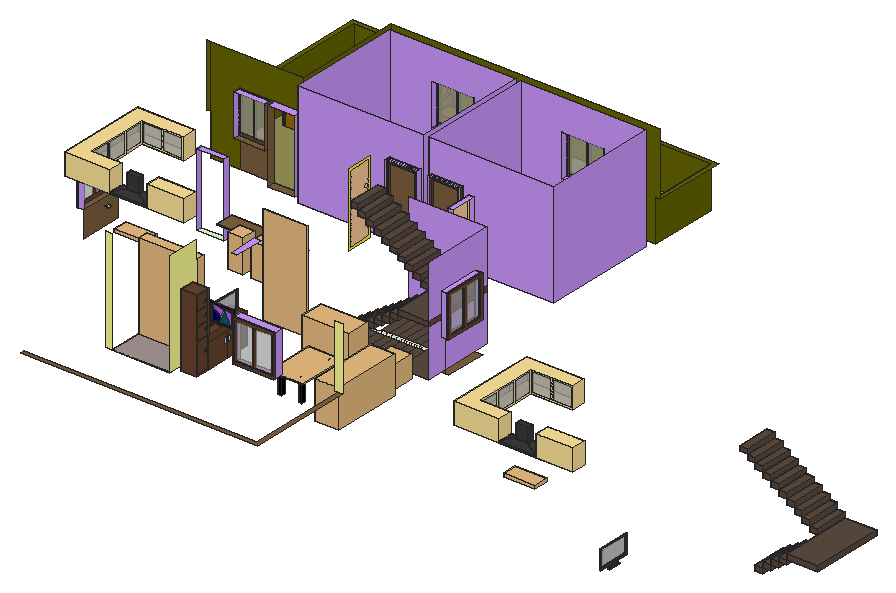
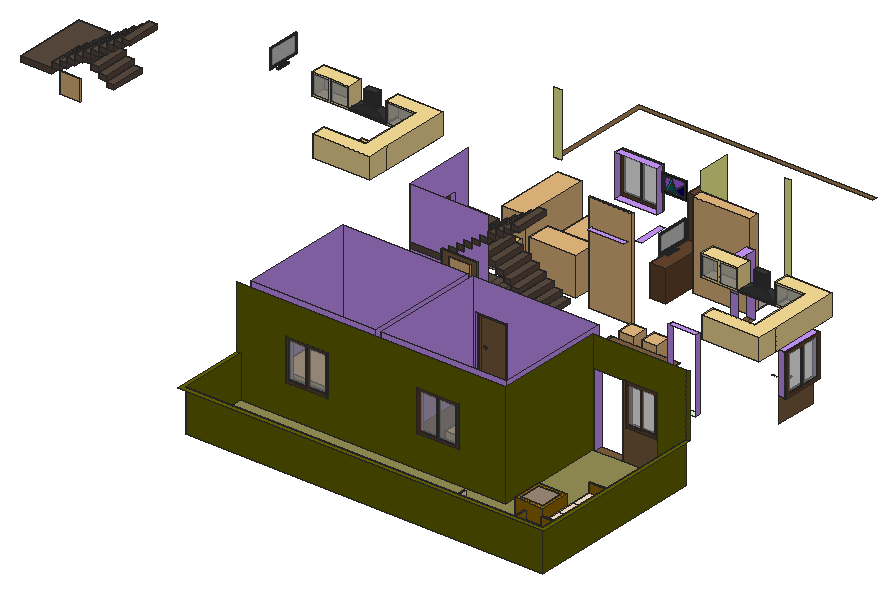
# SketchUp Ruby script. Lengths in inches.
U = 1.inch
M = Sketchup.active_model
def pt(a) = Geom::Point3d.new(a.map { |v| v * U })
def face(e, loops, mat)
  f = e.add_face(loops[0].map { |a| pt(a) })
  loops[1..].each { |l| e.add_face(l.map { |a| pt(a) }).erase! }
  f.material = f.back_material = mat if mat
  f
end
# faces: each face lists its corners as indices into pts; further lists are holes
def faces(e, pts, list, mat = nil) = list.each { |f| face(e, (f[0].is_a?(Array) ? f : [f]).map { |l| l.map { |i| pts[i] } }, mat) }
# xy, xz, yz: faces in a plane at the given z, y or x. An outline is a flat list of corners, or four numbers for a rectangle; further outlines are holes
def ring(l) = l.size == 4 ? [[l[0], l[1]], [l[2], l[1]], [l[2], l[3]], [l[0], l[3]]] : l.each_slice(2).to_a
def flat(e, list, mat, &to3) = list.each { |f| face(e, (f[0].is_a?(Array) ? f : [f]).map { |l| ring(l).map { |u, v| to3.(u, v) } }, mat) }
def xy(e, z, list, mat = nil) = flat(e, list, mat) { |x, y| [x, y, z] }
def xz(e, y, list, mat = nil) = flat(e, list, mat) { |x, z| [x, y, z] }
def yz(e, x, list, mat = nil) = flat(e, list, mat) { |y, z| [x, y, z] }
def lines(e, pts, list) = list.each { |a, b| e.add_line(pt(pts[a]), pt(pts[b])) }
# prism: a flat outline (further loops are holes) pulled along v
def prism(e, loops, v, mat = nil)
  f = face(e, loops, mat); d = Geom::Vector3d.new(v.map { |x| x * U })
  f.pushpull(f.normal.samedirection?(d) ? d.length : -d.length)
end
def box(e, o, s, mat = nil) = prism(e, [[o, [o[0] + s[0], o[1], o[2]], [o[0] + s[0], o[1] + s[1], o[2]], [o[0], o[1] + s[1], o[2]]]], [0, 0, s[2]], mat)
def at(x, y, z, deg = 0) = Geom::Transformation.translation(pt([x, y, z])) * Geom::Transformation.rotation(ORIGIN, Z_AXIS, deg.degrees)
def axes(o, x, y, z) = Geom::Transformation.new([*x, 0, *y, 0, *z, 0, *pt(o).to_a, 1])
def part(name) = M.definitions.add(name)
# library, detail: a bought-in or finely detailed component or shape, given as its bounding box
def library(name, o, s) = part(name).tap { |d| box(d.entities, o, s) }
def detail(e, o, s) = box(e.add_group.entities, o, s)
def put(e, d, t, mat = nil) = e.add_instance(d, t).tap { |i| i.material = mat if mat }
def group(e, t, mat = nil) = e.add_group.tap { |g| g.transformation = t; g.material = mat if mat }.entities
root = M.entities
M.materials.add("C01_Vanilla_Cream").color = [255, 230, 206]
M.materials.add("C02_Golden_Beige").color = [255, 205, 155]
M.materials.add("D02_Buttercup_Glow").color = [255, 229, 155]
M.materials.add("D07_Ochre_Flame").color = [153, 107, 0]
M.materials.add("E01_Mint_Frost").color = [255, 255, 204]
M.materials.add("E02_Pale_Lime").color = [255, 255, 153]
M.materials.add("E04_Green_Bloom").color = [255, 255, 49]
M.materials.add("E08_Lime_Depth").color = [102, 102, 0]
M.materials.add("F06_Grassy_Shade").color = [102, 204, 0]
M.materials.add("G07_Jungle_Burst").color = [0, 153, 0]
M.materials.add("Glass_Mirror_01").color = [185, 185, 185]
M.materials["Glass_Mirror_01"].alpha = 0.91
M.materials.add("Glass_Mirror_2").color = [185, 185, 185]
M.materials["Glass_Mirror_2"].alpha = 0.8
M.materials.add("Glass_Mirror_3").color = [185, 185, 185]
M.materials["Glass_Mirror_3"].alpha = 0.65
M.materials.add("Glass_Mirror_4").color = [185, 185, 185]
M.materials["Glass_Mirror_4"].alpha = 0.68
M.materials.add("Glass_Sky Reflection_01").color = [126, 138, 183]
M.materials["Glass_Sky Reflection_01"].alpha = 0.25
M.materials.add("H06_Ocean_Depth").color = [0, 204, 204]
M.materials.add("H08_Emerald_Abyss").color = [0, 102, 102]
M.materials.add("I03_Bluebell_Mist").color = [101, 101, 255]
M.materials.add("I08_Inkstorm").color = [0, 0, 102]
M.materials.add("J02_Lavender_Veil").color = [204, 153, 255]
M.materials.add("J03_Orchid_Glow").color = [178, 101, 255]
M.materials.add("K02_Rosy_Glow").color = [255, 153, 255]
M.materials.add("M07_Charcoal_Gleam").color = [58, 58, 58]
M.materials.add("M09_Shadow_Night").color = [0, 0, 0]
M.materials.add("Marble_01_1K").color = [230, 255, 211]
M.materials.add("Marble_03_1K").color = [175, 182, 201]
M.materials.add("Marble_06_1K").color = [165, 150, 147]
M.materials.add("Marble_07_1K").color = [36, 34, 36]
M.materials.add("Marble_20_1K").color = [172, 173, 182]
M.materials.add("Metal_06_1K").color = [238, 236, 231]
M.materials.add("Plaster_02_1K").color = [157, 140, 119]
M.materials.add("Plywood_01_1K").color = [125, 96, 64]
M.materials.add("Soil_04_1K").color = [152, 146, 88]
M.materials.add("Wood_Floor_12_1K").color = [92, 75, 65]
M.materials.add("Wood_Veneer_15_1K").color = [103, 69, 45]
c1 = part("Group\#70")
box(c1.entities,[0,0,0],[9,39,6],"Wood_Floor_12_1K")
c2 = part("Group\#38")
xy(c2.entities,0,[[67.3125,0,69.625,27.1875],[-2.33,24.1875,67.3125,27.1875]],"D07_Ochre_Flame")
xy(c2.entities,18.3125,[[0,0,22.82,24.1875],[22.82,0,45.07,24.1875],[45.07,0,67.3125,24.1875]],"C01_Vanilla_Cream")
xy(c2.entities,24.5625,[[67.3125,0,69.625,27.1875]],"D07_Ochre_Flame")
xy(c2.entities,28.6875,[[-2.33,0,0,24.1875]],"D07_Ochre_Flame")
xy(c2.entities,33.375,[[-2.33,24.1875,67.3125,27.1875]],"D07_Ochre_Flame")
xz(c2.entities,0,[[0,0,22.82,18.3125],[22.82,0,45.07,18.3125],[45.07,0,67.3125,18.3125]],"C01_Vanilla_Cream")
xz(c2.entities,0,[[-2.33,0,0,28.6875],[67.3125,0,69.625,24.5625]],"D07_Ochre_Flame")
xz(c2.entities,24.1875,[[-2.33,0,67.3125,0,67.3125,18.3125,0,18.3125,0,28.6875,-2.33,28.6875],[0,18.3125,22.82,33.375],[22.82,18.3125,45.07,33.375],[45.07,18.3125,67.3125,33.375],[-2.33,28.6875,0,33.375]],"D07_Ochre_Flame")
xz(c2.entities,27.1875,[[-2.33,0,67.3125,33.375],[67.3125,0,69.625,24.5625]],"D07_Ochre_Flame")
yz(c2.entities,-2.33,[[0,0,24.1875,28.6875],[24.1875,0,27.1875,33.375]],"D07_Ochre_Flame")
yz(c2.entities,0,[[0,18.3125,24.1875,28.6875]],"D07_Ochre_Flame")
yz(c2.entities,67.3125,[[0,0,24.1875,18.3125],[0,18.3125,24.1875,24.5625]],"C01_Vanilla_Cream")
yz(c2.entities,67.3125,[[24.1875,0,27.1875,24.5625],[24.1875,24.5625,27.1875,33.375]],"D07_Ochre_Flame")
yz(c2.entities,69.625,[[0,0,27.1875,24.5625]],"D07_Ochre_Flame")
c3 = part("Group\#43")
box(c3.entities,[0,0,0],[1,4.5625,0.25],"Metal_06_1K")
c4 = part("Group\#42")
xy(c4.entities,0,[[0,-1.93,40.35,0],[0,0,40.35,21.25]],"Plywood_01_1K")
xy(c4.entities,25.125,[[0,0,40.35,21.25]],"Marble_07_1K")
xy(c4.entities,25.1875,[[20.85,8.75,21.39,8.86,21.89,9.11,22.3,9.47,22.61,9.94,22.79,10.46,22.82,11.01,22.71,11.56,22.47,12.06,22.1,12.47,21.64,12.78,21.11,12.96,20.56,12.99,20.01,12.88,19.52,12.63,19.1,12.27,18.79,11.81,18.62,11.28,18.58,10.73,18.69,10.18,18.9375,9.69,19.31,9.27,19.77,8.96,20.29,8.79]],"M09_Shadow_Night")
xy(c4.entities,25.1875,[[[8.8,4,31.8,17.68],[20.85,8.75,20.29,8.79,19.77,8.96,19.31,9.27,18.9375,9.69,18.69,10.18,18.58,10.73,18.62,11.28,18.79,11.81,19.1,12.27,19.52,12.63,20.01,12.88,20.56,12.99,21.11,12.96,21.64,12.78,22.1,12.47,22.47,12.06,22.71,11.56,22.82,11.01,22.79,10.46,22.61,9.94,22.3,9.47,21.89,9.11,21.39,8.86]]],"Marble_07_1K")
xy(c4.entities,26,[[0,-1.93,40.35,0]],"Plywood_01_1K")
xy(c4.entities,26.5625,[[[0,0,40.35,21.25],[8.8,4,31.8,17.68]]],"Marble_07_1K")
xy(c4.entities,71.66,[[0,-1.93,40.35,0]],"Plywood_01_1K")
xz(c4.entities,-1.93,[[0,0,40.35,26],[0,26,40.35,71.66]],"Plywood_01_1K")
xz(c4.entities,0,[[0,25.125,40.35,26],[0,26,40.35,26.5625]],"Marble_07_1K")
xz(c4.entities,0,[[0,0,40.35,25.125],[0,26.5625,40.35,71.66]],"Plywood_01_1K")
xz(c4.entities,4,[[8.8,25.1875,31.8,26.5625]],"Marble_07_1K")
xz(c4.entities,17.68,[[8.8,25.1875,31.8,26.5625]],"Marble_07_1K")
xz(c4.entities,21.25,[[0,25.125,40.35,26.5625]],"Marble_07_1K")
xz(c4.entities,21.25,[[0,0,20.17,21],[20.17,0,40.35,21],[0,21,40.35,25.125]],"Plywood_01_1K")
yz(c4.entities,0,[[0,25.125,21.25,26.5625]],"Marble_07_1K")
yz(c4.entities,0,[[-1.93,0,0,26],[0,0,21.25,25.125],[-1.93,26,0,71.66]],"Plywood_01_1K")
yz(c4.entities,8.8,[[4,25.1875,17.68,26.5625]],"Marble_07_1K")
yz(c4.entities,31.8,[[4,25.1875,17.68,26.5625]],"Marble_07_1K")
yz(c4.entities,40.35,[[0,25.125,21.25,26.5625]],"Marble_07_1K")
yz(c4.entities,40.35,[[-1.93,0,0,26],[0,0,21.25,25.125],[-1.93,26,0,71.66]],"Plywood_01_1K")
put(c4.entities,c3,axes([22.63,21.25,13.17],[-1,0,0],[0,0,1],[0,1,0]))
put(c4.entities,c3,axes([18.69,21.25,13.17],[-1,0,0],[0,0,1],[0,1,0]))
put(c4.entities,c3,axes([22.61,21.25,24.2],[0,0,-1],[-1,0,0],[0,1,0]))
c5 = part("Group\#15")
box(c5.entities,[0,0,0],[4,4,24])
c6 = part("Group\#47")
box(c6.entities,[0,0,0],[65.6875,38.91,0.4375],"Marble_06_1K")
c7 = part("Group\#10")
detail(c7.entities,[0,-4,0],[28,80,43.625])
c8 = part("Group\#14")
box(c8.entities,[0,0,0],[4,4,24])
c9 = part("Group\#29")
box(c9.entities,[0,0,0],[20.5,20.5,18],"Wood_Veneer_15_1K")
c10 = part("Group\#11")
detail(c10.entities,[0,0,0],[24,24,25.375])
c11 = part("Group\#12")
detail(c11.entities,[-3,0,0],[54,27,43.625])
c12 = part("Group\#50")
xy(c12.entities,0,[[0,39,81,39,81,45,27,45,27,43,79,43,79,41,0,41]],"Metal_06_1K")
xy(c12.entities,0,[[9,0,18,39],[18,0,27,39],[27,0,36,39],[36,0,45,39],[45,0,54,39],
  [54,0,63,39],[63,0,72,39],[72,0,81,39],[81,0,117,84],[27,45,36,84],
  [36,45,45,84],[45,45,54,84],[54,45,63,84],[63,45,72,84],[72,45,81,84]],"Wood_Floor_12_1K")
put(c12.entities,c1,at(0,0,0))
put(c12.entities,c1,at(9,0,6))
put(c12.entities,c1,at(18,0,12))
put(c12.entities,c1,at(27,0,18))
put(c12.entities,c1,at(36,0,24))
put(c12.entities,c1,at(45,0,30))
put(c12.entities,c1,at(54,0,36))
put(c12.entities,c1,at(63,0,42))
put(c12.entities,c1,at(72,0,48))
g1 = group(c12.entities,at(81,0,54))
box(g1,[0,0,0],[36,84,6],"Wood_Floor_12_1K")
put(c12.entities,c1,at(72,45,60))
put(c12.entities,c1,at(63,45,66))
put(c12.entities,c1,at(54,45,72))
put(c12.entities,c1,at(45,45,78))
put(c12.entities,c1,at(36,45,84))
put(c12.entities,c1,at(27,45,90))
put(c12.entities,c1,at(18,45,96))
put(c12.entities,c1,at(9,45,102))
put(c12.entities,c1,at(0,45,108))
put(c12.entities,c1,at(-9,45,114))
c13 = part("Group\#51")
xy(c13.entities,0,[[0,39,81,39,81,45,27,45,27,43,79,43,79,41,0,41]],"Metal_06_1K")
xy(c13.entities,0,[[0,0,9,39],[9,0,18,39],[18,0,27,39],[27,0,36,39],[36,0,45,39],
  [45,0,54,39],[54,0,63,39],[63,0,72,39],[72,0,81,39],[81,0,117,84],
  [27,45,36,84],[36,45,45,84],[45,45,54,84],[54,45,63,84],[63,45,72,84],
  [72,45,81,84]],"Wood_Floor_12_1K")
c14 = library("Group\#63",[-3.99,-1.7,0],[49.63,1.7,114.25])
c15 = part("Group\#41")
xy(c15.entities,0,[[[0,0,32.5625,34],[3.65,3.65,28.91,30.35]]],"D07_Ochre_Flame")
xy(c15.entities,18.3125,[[[0,0,32.5625,34],[3.65,3.65,28.91,30.35]]],"D07_Ochre_Flame")
xy(c15.entities,18.3125,[[3.65,3.65,28.91,30.35]],"Plaster_02_1K")
xz(c15.entities,0,[[0,0,32.5625,18.3125]],"D07_Ochre_Flame")
xz(c15.entities,3.65,[[3.65,0,28.91,18.3125]],"D07_Ochre_Flame")
xz(c15.entities,30.35,[[3.65,0,28.91,18.3125]],"D07_Ochre_Flame")
xz(c15.entities,34,[[0,0,32.5625,18.3125]],"D07_Ochre_Flame")
yz(c15.entities,0,[[0,0,34,18.3125]],"D07_Ochre_Flame")
yz(c15.entities,3.65,[[3.65,0,30.35,18.3125]],"D07_Ochre_Flame")
yz(c15.entities,28.91,[[3.65,0,30.35,18.3125]],"D07_Ochre_Flame")
yz(c15.entities,32.5625,[[0,0,34,18.3125]],"D07_Ochre_Flame")
c16 = part("Group\#16")
box(c16.entities,[0,0,0],[4,4,24])
c17 = part("Group\#9")
box(c17.entities,[0,0,0],[0.75,3.75,0.1875],"Metal_06_1K")
c18 = part("Group\#2")
xy(c18.entities,0,[[0,-16.81,18.0625,0],[0,0,18.0625,55.25]],"Wood_Veneer_15_1K")
xy(c18.entities,36,[[0,0,18.0625,55.25]],"Wood_Veneer_15_1K")
xy(c18.entities,84,[[0,-16.81,18.0625,0]],"Wood_Veneer_15_1K")
xz(c18.entities,-16.81,[[0,0,18.0625,84]],"Wood_Veneer_15_1K")
xz(c18.entities,0,[[0,0,18.0625,36],[0,36,18.0625,84]],"Wood_Veneer_15_1K")
xz(c18.entities,55.25,[[0,0,18.0625,36]],"Wood_Veneer_15_1K")
yz(c18.entities,0,[[-16.81,0,0,84],[0,0,55.25,36]],"Wood_Veneer_15_1K")
yz(c18.entities,18.0625,[[[-16.81,0,0,84],[-14.81,2,-2,82]],[0,0,27.625,27.91],[27.625,0,55.25,27.91],[-14.81,2,-2,35],[0,27.91,55.25,36],
  [-14.81,35,-2,36],[-14.81,36,-2,50.3125],[-14.81,50.3125,-2,51.3125],[-14.81,51.3125,-2,65.85],[-14.81,65.85,-2,66.85],
  [-14.81,66.85,-2,82]],"Wood_Veneer_15_1K")
g2 = group(c18.entities,at(18.0625,23.18,16.77))
box(g2,[0,0,0],[0.2,1.5,6.25],"Metal_06_1K")
g3 = group(c18.entities,at(18.0625,29.74,16.77))
box(g3,[0,0,0],[0.2,1.5,6.25],"Metal_06_1K")
put(c18.entities,c17,axes([18.0625,-4.49,72.03],[0,1,0],[0,0,1],[1,0,0]))
put(c18.entities,c17,axes([18.0625,-4.49,57.4],[0,1,0],[0,0,1],[1,0,0]))
put(c18.entities,c17,axes([18.0625,-4.49,42.9],[0,1,0],[0,0,1],[1,0,0]))
put(c18.entities,c17,axes([18.0625,-4.49,20.71],[0,1,0],[0,0,1],[1,0,0]))
c19 = library("Group\#27",[0,0,0],[94.3125,62.5,20])
c20 = part("Group\#17")
box(c20.entities,[0,0,0],[4,4,24])
c21 = library("Group\#36",[0,0,0],[17.25,17.25,38])
c22 = part("Group\#40")
box(c22.entities,[0,4,0],[19.9375,19.25,18.3125],"D07_Ochre_Flame")
c23 = library("Group\#54",[0,-12,0],[65.6875,12,119.5625])
c24 = part("Group\#61")
prism(c24.entities,[[[0.51,0.51,0],[0.23,0.875,0],[0.06,1.3,0],[0,1.75,0],[0.06,2.2,0],[0.23,2.625,0],[0.51,2.99,0],[0.875,3.27,0],[1.3,3.44,0],[1.75,3.5,0],[2.2,3.44,0],[2.625,3.27,0],[2.99,2.99,0],[3.27,2.625,0],[3.44,2.2,0],[3.5,1.75,0],[3.44,1.3,0],[3.27,0.875,0],[2.99,0.51,0],[2.625,0.23,0],[2.2,0.06,0],[1.75,0,0],[1.3,0.06,0],[0.875,0.23,0]]],[0,0,0.625],"Metal_06_1K")
c25 = part("Group\#59")
xy(c25.entities,0,[[0,-2,36,0]],"Wood_Veneer_15_1K")
xy(c25.entities,3,[[3,-0.5,33,0]])
xy(c25.entities,3,[[3,-2,33,-0.5]],"Wood_Veneer_15_1K")
xy(c25.entities,81,[[3,-0.5,33,0]])
xy(c25.entities,81,[[3,-2,33,-0.5]],"Wood_Veneer_15_1K")
xy(c25.entities,84,[[0,-2,36,0]],"Wood_Veneer_15_1K")
xz(c25.entities,-2,[[[0,0,36,84],[3,3,33,81]]],"Wood_Veneer_15_1K")
xz(c25.entities,-0.5,[[3,3,33,81]])
xz(c25.entities,0,[[[0,0,36,84],[3,3,33,81]]],"Wood_Veneer_15_1K")
yz(c25.entities,0,[[-2,0,0,84]],"Wood_Veneer_15_1K")
yz(c25.entities,3,[[-0.5,3,0,81]])
yz(c25.entities,3,[[-2,3,-0.5,81]],"Wood_Veneer_15_1K")
yz(c25.entities,33,[[-0.5,3,0,81]])
yz(c25.entities,33,[[-2,3,-0.5,81]],"Wood_Veneer_15_1K")
yz(c25.entities,36,[[-2,0,0,84]],"Wood_Veneer_15_1K")
put(c25.entities,c24,axes([25.79,-0.5,47.4],[1,0,0],[0,0,1],[0,-1,0]))
put(c25.entities,c24,axes([57.22,-0.5,47.4],[1,0,0],[0,0,1],[0,-1,0]))
c26 = part("Group\#60")
xy(c26.entities,0,[[0,-2,36,0]],"Wood_Veneer_15_1K")
xy(c26.entities,3,[[3,-0.5,33,0]])
xy(c26.entities,3,[[3,-2,33,-0.5]],"Wood_Veneer_15_1K")
xy(c26.entities,81,[[3,-0.5,33,0]])
xy(c26.entities,81,[[3,-2,33,-0.5]],"Wood_Veneer_15_1K")
xy(c26.entities,84,[[0,-2,36,0]],"Wood_Veneer_15_1K")
xz(c26.entities,-2,[[[0,0,36,84],[3,3,33,81]]],"Wood_Veneer_15_1K")
xz(c26.entities,-0.5,[[3,3,33,81]])
xz(c26.entities,0,[[[0,0,36,84],[3,3,33,81]]],"Wood_Veneer_15_1K")
yz(c26.entities,0,[[-2,0,0,84]],"Wood_Veneer_15_1K")
yz(c26.entities,3,[[-0.5,3,0,81]])
yz(c26.entities,3,[[-2,3,-0.5,81]],"Wood_Veneer_15_1K")
yz(c26.entities,33,[[-0.5,3,0,81]])
yz(c26.entities,33,[[-2,3,-0.5,81]],"Wood_Veneer_15_1K")
yz(c26.entities,36,[[-2,0,0,84]],"Wood_Veneer_15_1K")
c27 = part("Group\#62")
yz(c27.entities,-0.625,[[5.65,55.09,5.28,55.14,4.93,55.28,4.64,55.51,4.41,55.81,4.26,56.15,4.22,56.53,4.26,56.9,4.41,57.25,4.64,57.54,4.93,57.77,5.28,57.92,5.65,57.96,6.03,57.92,6.37,57.77,6.67,57.54,6.9,57.25,7.04,56.9,7.09,56.53,7.04,56.15,6.9,55.81,6.67,55.51,6.37,55.28,6.03,55.14]],"Metal_06_1K")
yz(c27.entities,0,[[[2.8125,2.8125,27.1875,81.1875],[5.65,55.09,6.03,55.14,6.37,55.28,6.67,55.51,6.9,55.81,7.04,56.15,7.09,56.53,7.04,56.9,6.9,57.25,6.67,57.54,6.37,57.77,6.03,57.92,5.65,57.96,5.28,57.92,4.93,57.77,4.64,57.54,4.41,57.25,4.26,56.9,4.22,56.53,4.26,56.15,4.41,55.81,4.64,55.51,4.93,55.28,5.28,55.14]]],"C02_Golden_Beige")
yz(c27.entities,0,[[[0,0,30,84],[2.8125,2.8125,27.1875,81.1875]]],"E04_Green_Bloom")
p = [[0,5.28,55.14],[0,4.93,55.28],[-0.625,4.93,55.28],[-0.625,5.28,55.14],[0,5.65,55.09],[-0.625,5.65,55.09],
  [0,6.03,55.14],[-0.625,6.03,55.14],[0,6.37,55.28],[-0.625,6.37,55.28],[0,4.64,55.51],[-0.625,4.64,55.51],
  [0,6.67,55.51],[-0.625,6.67,55.51],[0,4.41,55.81],[-0.625,4.41,55.81],[0,6.9,55.81],[-0.625,6.9,55.81],
  [0,4.26,56.15],[-0.625,4.26,56.15],[0,7.04,56.15],[-0.625,7.04,56.15],[0,4.22,56.53],[-0.625,4.22,56.53],
  [0,7.09,56.53],[-0.625,7.09,56.53],[0,4.26,56.9],[-0.625,4.26,56.9],[0,7.04,56.9],[-0.625,7.04,56.9],
  [0,4.41,57.25],[-0.625,4.41,57.25],[0,6.9,57.25],[-0.625,6.9,57.25],[0,4.64,57.54],[-0.625,4.64,57.54],
  [0,6.67,57.54],[-0.625,6.67,57.54],[0,4.93,57.77],[-0.625,4.93,57.77],[0,6.37,57.77],[-0.625,6.37,57.77],
  [0,5.28,57.92],[-0.625,5.28,57.92],[0,6.03,57.92],[-0.625,6.03,57.92],[0,5.65,57.96],[-0.625,5.65,57.96]]
faces(c27.entities,p,[[0,1,2,3],[4,0,3,5],[6,4,5,7],[8,6,7,9],[1,10,11,2],[12,8,9,13],[10,14,15,11],[16,12,13,17],
  [14,18,19,15],[20,16,17,21],[18,22,23,19],[24,20,21,25],[22,26,27,23],[28,24,25,29],[26,30,31,27],[32,28,29,33],
  [30,34,35,31],[36,32,33,37],[34,38,39,35],[40,36,37,41],[38,42,43,39],[44,40,41,45],[42,46,47,43],[46,44,45,47]],"Metal_06_1K")
c28 = library("Group\#28",[0,0,0],[94.3125,62.5,20])
c29 = part("Group\#8")
g4 = group(c29.entities,at(0.75,15.42,1.1875),"M07_Charcoal_Gleam")
prism(g4,[[[1.25,5.68,0],[1.25,0.93,0],[0.46,0.6,0],[0.3125,0.54,0],[0.18,0.44,0],[0.08,0.3125,0],[0.02,0.16,0],[0,0,0],[0,6.6875,0],[0.02,6.53,0],[0.08,6.375,0],[0.18,6.25,0],[0.3125,6.15,0],[0.46,6.08,0],[0.625,6.0625,0]]],[0,0,3.25])
g5 = group(c29.entities,at(0,11.83,0))
box(g5,[0,0,0],[2.8125,14.875,1.1875],"M07_Charcoal_Gleam")
g6 = group(c29.entities,at(2,0,4.4375))
xy(g6,0,[[-1,0,0,37.44]],"M07_Charcoal_Gleam")
xy(g6,21.9,[[-1,0,0,37.44]],"M07_Charcoal_Gleam")
xz(g6,0,[[-1,0,0,21.9]],"M07_Charcoal_Gleam")
xz(g6,37.44,[[-1,0,0,21.9]],"M07_Charcoal_Gleam")
yz(g6,-1,[[1.62,1.96,35.68,20.27]],"Glass_Mirror_01")
yz(g6,-1,[[[0,0,37.44,21.9],[1.62,1.96,35.68,20.27]]],"M07_Charcoal_Gleam")
yz(g6,0,[[[0,0,37.44,21.9],[1.62,1.96,35.68,20.27]]],"M07_Charcoal_Gleam")
p = [[0,35.68,20.27],[-1,35.68,20.27],[0,1.62,20.27],[-1,1.62,20.27],[0,35.68,1.96],[-1,35.68,1.96],
  [0,1.62,1.96],[-1,1.62,1.96]]
lines(g6,p,[[0,1],[2,3],[4,5],[6,7]])
c30 = library("Group\#23",[0,0,0],[35.8125,17,3.54])
c31 = part("Group\#44")
detail(c31.entities,[0,0,0],[24,1.25,24])
c32 = part("Group\#13")
detail(c32.entities,[-5.9375,-5.9375,0],[39.25,56.8125,1])
c33 = part("Group\#57")
xy(c33.entities,0,[[0,-2,48,0]],"Wood_Veneer_15_1K")
xy(c33.entities,3,[[3,-2,23,0],[25,-2,45,0]],"Wood_Veneer_15_1K")
xy(c33.entities,45,[[3,-2,23,0],[25,-2,45,0]],"Wood_Veneer_15_1K")
xy(c33.entities,48,[[0,-2,48,0]],"Wood_Veneer_15_1K")
xz(c33.entities,-2,[[[0,0,48,48],[25,3,45,45],[3,3,23,45]]],"Wood_Veneer_15_1K")
xz(c33.entities,0,[[3,3,23,45],[25,3,45,45]],"Glass_Mirror_4")
xz(c33.entities,0,[[[0,0,48,48],[25,3,45,45],[3,3,23,45]]],"Wood_Veneer_15_1K")
yz(c33.entities,0,[[-2,0,0,48]],"Wood_Veneer_15_1K")
yz(c33.entities,3,[[-2,3,0,45]],"Wood_Veneer_15_1K")
yz(c33.entities,23,[[-2,3,0,45]],"Wood_Veneer_15_1K")
yz(c33.entities,25,[[-2,3,0,45]],"Wood_Veneer_15_1K")
yz(c33.entities,45,[[-2,3,0,45]],"Wood_Veneer_15_1K")
yz(c33.entities,48,[[-2,0,0,48]],"Wood_Veneer_15_1K")
c34 = library("Group\#24",[0,0,0],[4.375,4.375,0.1875])
c35 = part("Group\#56")
xy(c35.entities,0,[[0,0,2,48]],"Wood_Veneer_15_1K")
xy(c35.entities,3,[[0,3,2,23],[0,25,2,45]],"Wood_Veneer_15_1K")
xy(c35.entities,45.04,[[0,3,2,23],[0,25,2,45]],"Wood_Veneer_15_1K")
xy(c35.entities,48.04,[[0,0,2,48]],"Wood_Veneer_15_1K")
xz(c35.entities,0,[[0,0,2,48.04]],"Wood_Veneer_15_1K")
xz(c35.entities,3,[[0,3,2,23.02],[0,23.02,2,25.02],[0,25.02,2,45.04]],"Wood_Veneer_15_1K")
xz(c35.entities,23,[[0,3,2,23.02],[0,23.02,2,25.02],[0,25.02,2,45.04]],"Wood_Veneer_15_1K")
xz(c35.entities,25,[[0,3,2,23.02],[0,23.02,2,25.02],[0,25.02,2,45.04]],"Wood_Veneer_15_1K")
xz(c35.entities,45,[[0,3,2,23.02],[0,23.02,2,25.02],[0,25.02,2,45.04]],"Wood_Veneer_15_1K")
xz(c35.entities,48,[[0,0,2,48.04]],"Wood_Veneer_15_1K")
yz(c35.entities,0,[[3,3,23,45.04],[25,3,45,45.04]],"Glass_Mirror_3")
yz(c35.entities,0,[[[0,0,48,48.04],[3,3,23,45.04],[25,3,45,45.04]]],"Wood_Veneer_15_1K")
yz(c35.entities,2,[[[0,0,48,48.04],[3,3,23,45.04],[25,3,45,45.04]]],"Wood_Veneer_15_1K")
c36 = part("Group\#37")
xy(c36.entities,0,[[0,0,52.33,16.76],[94.85,0,137.375,16.76],[0,16.76,0,104.9375,66.09,104.9375,66.09,88.6875,18.42,88.6875,18.42,16.76]],"D02_Buttercup_Glow")
xy(c36.entities,0,[[52.33,0,94.85,16.76]],"M07_Charcoal_Gleam")
xy(c36.entities,24.5625,[[0,0,52.33,0,52.33,16.76,18.42,16.76,18.42,88.6875,66.09,88.6875,66.09,104.9375,0,104.9375],[94.85,0,137.375,16.76]],"D02_Buttercup_Glow")
xz(c36.entities,0,[[0,0,52.33,24.5625],[94.85,0,137.375,24.5625]],"D02_Buttercup_Glow")
xz(c36.entities,0,[[52.33,0,94.85,2.0625]],"M07_Charcoal_Gleam")
xz(c36.entities,16.76,[[[18.42,0,52.33,24.5625],[20.03,1.61,50.72,22.95]],[[94.85,0,116.11,24.5625],[96.47,1.61,114.5,22.95]],[[116.11,0,137.375,24.5625],[117.8125,1.7,135.68,22.87]]],"D02_Buttercup_Glow")
xz(c36.entities,16.76,[[20.03,1.61,50.72,22.95],[96.47,1.61,114.5,22.95],[117.8125,1.7,135.68,22.87]],"Glass_Mirror_2")
xz(c36.entities,16.76,[[52.33,0,94.85,2.0625]],"M07_Charcoal_Gleam")
xz(c36.entities,88.6875,[[[18.42,0,42.25,24.5625],[20.03,1.61,40.64,22.95]],[[42.25,0,66.09,24.5625],[43.87,1.61,64.48,22.95]]],"D02_Buttercup_Glow")
xz(c36.entities,88.6875,[[20.03,1.61,40.64,22.95],[43.87,1.61,64.48,22.95]],"Glass_Mirror_2")
xz(c36.entities,104.9375,[[0,0,66.09,24.5625]],"D02_Buttercup_Glow")
yz(c36.entities,0,[[0,0,80.9375,24.5625],[80.9375,0,104.9375,24.5625]],"D02_Buttercup_Glow")
yz(c36.entities,18.42,[[[16.76,0,40.76,24.5625],[18.37,1.61,39.15,22.95]],[[40.76,0,64.76,24.5625],[42.37,1.61,63.15,22.95]],[[64.76,0,88.6875,24.5625],[66.37,1.61,87.08,22.95]]],"D02_Buttercup_Glow")
yz(c36.entities,18.42,[[18.37,1.61,39.15,22.95],[42.37,1.61,63.15,22.95],[66.37,1.61,87.08,22.95]],"Glass_Mirror_2")
yz(c36.entities,52.33,[[0,2.0625,16.76,24.5625]],"D02_Buttercup_Glow")
yz(c36.entities,52.33,[[0,0,16.76,2.0625]],"M07_Charcoal_Gleam")
yz(c36.entities,66.09,[[88.6875,0,104.9375,24.5625]],"D02_Buttercup_Glow")
yz(c36.entities,94.85,[[0,2.0625,16.76,24.5625]],"D02_Buttercup_Glow")
yz(c36.entities,94.85,[[0,0,16.76,2.0625]],"M07_Charcoal_Gleam")
yz(c36.entities,137.375,[[0,0,16.76,24.5625]],"D02_Buttercup_Glow")
g7 = group(c36.entities,at(67.95,4.33,2.0625))
xy(g7,0,[[[-15.61,-4.33,26.91,12.43],[0,0,13.8125,6.75]],[0,0,13.8125,6.75]],"M07_Charcoal_Gleam")
xy(g7,6.25,[[0,0,13.8125,6.75]],"M07_Charcoal_Gleam")
xy(g7,22.5,[[0,0,13.8125,6.75]],"M07_Charcoal_Gleam")
xz(g7,0,[[0,0,13.8125,6.25],[0,6.25,13.8125,22.5]],"M07_Charcoal_Gleam")
xz(g7,6.75,[[0,0,13.8125,6.25],[0,6.25,13.8125,22.5]],"M07_Charcoal_Gleam")
yz(g7,0,[[0,0,6.75,6.25],[0,6.25,6.75,22.5]],"M07_Charcoal_Gleam")
yz(g7,13.8125,[[0,0,6.75,6.25],[0,6.25,6.75,22.5]],"M07_Charcoal_Gleam")
p = [[-15.61,-4.33,0],[0,0,6.25],[0,6.75,6.25],[-15.61,12.43,0],[26.91,-4.33,0],[13.8125,0,6.25],
  [26.91,12.43,0],[13.8125,6.75,6.25]]
faces(g7,p,[[0,1,2,3],[4,5,1,0],[4,6,7,5],[3,2,7,6]],"M07_Charcoal_Gleam")
c37 = part("Group\#66")
xy(c37.entities,0,[[0,0,27.25,1]],"M09_Shadow_Night")
xy(c37.entities,1.6,[[1.6,0.125,25.65,1]])
xy(c37.entities,1.6,[[1.6,0,25.65,0.125]],"M09_Shadow_Night")
xy(c37.entities,18.71,[[1.6,0.125,25.65,1]])
xy(c37.entities,18.71,[[1.6,0,25.65,0.125]],"M09_Shadow_Night")
xy(c37.entities,20.3125,[[0,0,27.25,1]],"M09_Shadow_Night")
xz(c37.entities,0,[[[0,0,27.25,20.3125],[1.6,1.6,25.65,18.71]]],"M09_Shadow_Night")
xz(c37.entities,0.125,[[[25.65,15.53,11.53,18.71,25.65,18.71],[25.29,15.97,25.29,18.36,14.71,18.36]]],"F06_Grassy_Shade")
xz(c37.entities,0.125,[[25.29,15.97,14.71,18.36,25.29,18.36]],"G07_Jungle_Burst")
xz(c37.entities,0.125,[[[10.47,1.6,12.94,7.09,17,16.09,23.34,1.6],[11.43,2.22,22.39,2.22,16.99,14.5625,13.51,6.83]]],"H06_Ocean_Depth")
xz(c37.entities,0.125,[[11.43,2.22,13.51,6.83,16.99,14.5625,22.39,2.22]],"H08_Emerald_Abyss")
xz(c37.entities,0.125,[[[1.6,1.6,1.6,15.53,12.94,7.09,10.47,1.6],[2.22,2.22,10.07,2.22,12.18,6.89,2.22,14.29]]],"I03_Bluebell_Mist")
xz(c37.entities,0.125,[[2.22,2.22,2.22,14.29,12.18,6.89,10.07,2.22]],"I08_Inkstorm")
xz(c37.entities,0.125,[[23.64,2.06,17.1,16.99,25.19,15.16,25.19,2.06],[12.76,7.79,2.06,15.75,2.06,18.25,11.48,18.25,16.92,17.03]],"J03_Orchid_Glow")
xz(c37.entities,0.125,[[[23.34,1.6,17,16.09,12.94,7.09,1.6,15.53,1.6,18.71,11.53,18.71,25.65,15.53,25.65,1.6],[12.76,7.79,16.92,17.03,11.48,18.25,2.06,18.25,2.06,15.75],[23.64,2.06,25.19,2.06,25.19,15.16,17.1,16.99]]],"K02_Rosy_Glow")
xz(c37.entities,1,[[[0,0,27.25,20.3125],[1.6,1.6,25.65,18.71]]],"M09_Shadow_Night")
yz(c37.entities,0,[[0,0,1,20.3125]],"M09_Shadow_Night")
yz(c37.entities,1.6,[[0.125,1.6,1,18.71]])
yz(c37.entities,1.6,[[0,1.6,0.125,18.71]],"M09_Shadow_Night")
yz(c37.entities,25.65,[[0.125,1.6,1,18.71]])
yz(c37.entities,25.65,[[0,1.6,0.125,18.71]],"M09_Shadow_Night")
yz(c37.entities,27.25,[[0,0,1,20.3125]],"M09_Shadow_Night")
xy(root,36,[[1644.54,2081.58,1675.875,2087.58]],"Marble_01_1K")
xy(root,36,[[1888.04,2137.61,1894.04,2167.61]],"Marble_03_1K")
xy(root,36,[[1722.42,1862.58,1788.11,1901.49]],"Marble_20_1K")
xy(root,36,[[1713.42,1916.04,1717.92,1940.04],[1717.92,1916.04,1722.42,1940.04],[1978.04,2015.58,1987.04,2063.58],[1761.26,2060.28,1763.8,2081.58],[1644.54,2183.58,1675.875,2192.58]],"Plywood_01_1K")
xy(root,36,[[1571.73,2192.58,1678.04,2192.58,1678.04,2318.58,1982.36,2318.58,1982.36,2397.95,1571.73,2397.95]],"Soil_04_1K")
xy(root,36,[[1684.04,2177.58,1828.04,2309.58],[1834.04,2177.58,1978.04,2309.58]],"Wood_Floor_12_1K")
xy(root,36,[[1788.97,2171.58,1824.97,2177.58],[1837.82,2171.58,1873.82,2177.58]],"Wood_Veneer_15_1K")
xy(root,64.6875,[[1684.04,2060.28,1761.26,2081.58],[1761.26,2060.28,1763.8,2081.58]],"Plywood_01_1K")
xy(root,65.6875,[[1684.04,2060.28,1763.8,2081.58]],"Plywood_01_1K")
xy(root,66,[[1567.04,2005.11,1576.04,2053.11]],"Plywood_01_1K")
xy(root,72,[[1862.07,1862.58,1910.07,1871.58],[1882.04,2309.58,1930.04,2318.58]],"J02_Lavender_Veil")
xy(root,72,[[1978.04,2015.58,1987.04,2063.58],[1605.14,2183.58,1641.14,2192.58],[1732.04,2309.58,1780.04,2318.58]],"Plywood_01_1K")
xy(root,73,[[1579.51,2036.36,1597.51,2036.99]],"Metal_06_1K")
xy(root,84,[[1567.04,2192.58,1571.73,2192.58,1571.73,2397.95,1982.36,2397.95,1982.36,2318.58,1987.04,2318.58,1987.04,2402.64,1567.04,2402.64]],"E08_Lime_Depth")
xy(root,84,[[1714.42,1740.42,1987.04,1740.42,1987.04,1862.58,1982.36,1862.58,1982.36,1745.11,1714.42,1745.11]],"Plywood_01_1K")
xy(root,108,[[1713.42,1916.04,1722.42,1940.04]],"J02_Lavender_Veil")
xy(root,114,[[1567.04,2005.11,1576.04,2053.11]],"J02_Lavender_Veil")
xy(root,120,[[1862.07,1862.58,1910.07,1871.58],[1788.11,1951.47,1794.11,1985.89],[1798.45,1991.58,1840.09,1997.58],[1644.54,2081.58,1675.875,2087.58],[1888.04,2137.61,1894.04,2167.61],
  [1788.97,2171.58,1824.97,2177.58],[1837.82,2171.58,1873.82,2177.58],[1605.14,2183.58,1675.875,2192.58],[1732.04,2309.58,1780.04,2318.58],[1882.04,2309.58,1930.04,2318.58]],"J02_Lavender_Veil")
xy(root,120.0625,[[1641.14,2183.58,1644.54,2192.58]],"Plywood_01_1K")
xz(root,1862.58,[[1714.42,36.4375,1722.42,156],[1978.04,84,1987.04,156]],"E02_Pale_Lime")
xz(root,1916.04,[[1713.42,36,1722.42,108]],"J02_Lavender_Veil")
xz(root,1940.04,[[1713.42,36,1722.42,72],[1713.42,72,1722.42,108]],"J02_Lavender_Veil")
xz(root,2005.11,[[1567.04,66,1576.04,114]],"J02_Lavender_Veil")
xz(root,2015.58,[[1978.04,72,1978.04,120,1987.04,120.04,1987.04,72]],"J02_Lavender_Veil")
xz(root,2053.11,[[1567.04,66,1576.04,114]],"J02_Lavender_Veil")
xz(root,2060.28,[[1761.26,36,1763.8,64.6875],[1684.04,64.6875,1763.8,65.6875]],"Plywood_01_1K")
xz(root,2063.58,[[1978.04,72,1987.04,72,1987.04,120.04,1978.04,120]],"J02_Lavender_Veil")
xz(root,2081.58,[[1888.04,36,1978.04,156]],"J02_Lavender_Veil")
xz(root,2081.58,[[1761.26,36,1763.8,64.6875],[1684.04,64.6875,1763.8,65.6875]],"Plywood_01_1K")
xz(root,2137.61,[[1888.04,36,1894.04,120]],"J02_Lavender_Veil")
xz(root,2167.61,[[1888.04,36,1894.04,120]],"J02_Lavender_Veil")
xz(root,2177.58,[[1684.04,36,1684.04,156,1828.04,156,1828.04,36,1824.97,36,1824.97,120,1788.97,120,1788.97,36],[1834.04,36,1834.04,156,1978.04,156,1978.04,36,1873.82,36,1873.82,120,1837.82,120,1837.82,36]],"J02_Lavender_Veil")
xz(root,2183.58,[[1641.14,120,1644.54,120.0625]],"J02_Lavender_Veil")
xz(root,2192.58,[[1571.73,36,1571.73,156,1678.04,156,1678.04,36,1675.875,36,1675.875,120,1644.54,120,1644.54,120.0625,1641.14,120.0625,1641.14,120,1605.14,120,1605.14,36],[1567.04,84,1571.73,156]],"E08_Lime_Depth")
xz(root,2192.58,[[1641.14,120,1644.54,120.0625]],"J02_Lavender_Veil")
xz(root,2192.58,[[1605.14,36,1605.14,72,1641.14,72,1641.14,120,1644.54,120,1644.54,36]],"Plywood_01_1K")
xz(root,2309.58,[[[1684.04,36,1828.04,156],[1732.04,72,1780.04,120]],[[1834.04,36,1978.04,156],[1882.04,72,1930.04,120]]],"J02_Lavender_Veil")
xz(root,2318.58,[[[1678.04,36,1678.04,156,1987.04,156,1987.04,84,1982.36,84,1982.36,36],[1882.04,72,1930.04,120],[1732.04,72,1780.04,120]]],"E08_Lime_Depth")
xz(root,2397.95,[[1571.73,36,1982.36,84]],"E08_Lime_Depth")
yz(root,1571.73,[[2192.58,36,2397.95,84]],"E08_Lime_Depth")
yz(root,1576.04,[[2005.11,37,2053.11,66]],"Plywood_01_1K")
yz(root,1605.14,[[2183.58,72,2192.58,120]],"J02_Lavender_Veil")
yz(root,1641.14,[[2183.58,72,2192.58,120.0625]],"Plywood_01_1K")
yz(root,1644.54,[[2081.58,36,2087.58,120]],"J02_Lavender_Veil")
yz(root,1644.54,[[2183.58,36,2192.58,120.0625]],"Plywood_01_1K")
yz(root,1675.875,[[2081.58,36,2087.58,120],[2183.58,36,2192.58,120]],"J02_Lavender_Veil")
yz(root,1678.04,[[2192.58,36,2318.58,156]],"E08_Lime_Depth")
yz(root,1684.04,[[2177.58,36,2309.58,156]],"J02_Lavender_Veil")
yz(root,1684.04,[[2060.28,64.6875,2081.58,65.6875]],"Plywood_01_1K")
yz(root,1732.04,[[2309.58,72,2318.58,120]],"J02_Lavender_Veil")
yz(root,1761.26,[[2060.28,36,2081.58,64.6875]],"Plywood_01_1K")
yz(root,1763.8,[[2060.28,36,2081.58,64.6875],[2060.28,64.6875,2081.58,65.6875]],"Plywood_01_1K")
yz(root,1780.04,[[2309.58,72,2318.58,120]],"J02_Lavender_Veil")
yz(root,1788.11,[[1862.58,36,1862.58,156,1900.1875,156,1900.1875,135.24,1901.49,135.24,1901.49,36]],"E02_Pale_Lime")
yz(root,1788.97,[[2171.58,36,2177.58,120]],"J02_Lavender_Veil")
yz(root,1824.97,[[2171.58,36,2177.58,120]],"J02_Lavender_Veil")
yz(root,1828.04,[[2177.58,36,2309.58,156]],"J02_Lavender_Veil")
yz(root,1834.04,[[2177.58,36,2309.58,156]],"J02_Lavender_Veil")
yz(root,1837.82,[[2171.58,36,2177.58,120]],"J02_Lavender_Veil")
yz(root,1862.07,[[1862.58,72,1871.58,120]],"J02_Lavender_Veil")
yz(root,1873.82,[[2171.58,36,2177.58,120]],"J02_Lavender_Veil")
yz(root,1882.04,[[2309.58,72,2318.58,120]],"J02_Lavender_Veil")
yz(root,1910.07,[[1862.58,72,1871.58,120]],"J02_Lavender_Veil")
yz(root,1930.04,[[2309.58,72,2318.58,120]],"J02_Lavender_Veil")
yz(root,1978.04,[[[1997.58,36,2081.58,156],[2015.58,72,2063.58,120]],[2177.58,36,2309.58,156]],"J02_Lavender_Veil")
yz(root,1982.36,[[2318.58,36,2397.95,84]],"E08_Lime_Depth")
p = [[1987.04,2015.58,120.04],[1978.04,2015.58,120],[1978.04,2063.58,120],[1987.04,2063.58,120.04],[1982.54,2015.58,36],[1982.54,2015.58,72]]
faces(root,p,[[0,1,2,3]],"J02_Lavender_Veil")
lines(root,p,[[4,5]])
put(root,c1,at(2425.13,1907.85,36),"Plywood_01_1K")
put(root,c2,at(1611.81,2282.16,36,90.739),"Plywood_01_1K")
put(root,c4,at(1894.64,2089.5,36),"Plywood_01_1K")
put(root,c5,at(1912.35,1892.47,36),"M09_Shadow_Night")
put(root,c6,at(1722.42,1862.58,36),"Plywood_01_1K")
put(root,c7,at(1945.27,1879.05,36),"Plywood_01_1K")
put(root,c8,at(1889.29,1892.47,36),"M09_Shadow_Night")
put(root,c9,at(1952.64,2197.46,36),"E01_Mint_Frost")
put(root,c10,at(1941.19,1965.86,36),"Plywood_01_1K")
put(root,c11,at(1867.15,1958.1875,36),"Plywood_01_1K")
put(root,c12,at(1861.04,1997.58,36),"Plywood_01_1K")
put(root,c13,at(1861.04,1997.58,36),"Plywood_01_1K")
put(root,c14,at(1798.09,1991.58,36),"E02_Pale_Lime")
put(root,c15,at(1625.93,2295.69,36),"Plywood_01_1K")
put(root,c16,at(1889.29,1934.16,36),"M09_Shadow_Night")
put(root,c9,at(1952.64,2280.46,36),"E01_Mint_Frost")
put(root,c18,at(1794.11,1888.38,36),"Plywood_01_1K")
put(root,c19,at(1973.14,2280.46,36,-180),"Plywood_01_1K")
put(root,c20,at(1912.35,1934.16,36),"M09_Shadow_Night")
put(root,c21,at(1710.39,2043.07,36),"Plywood_01_1K")
put(root,c21,at(1736.76,2043.07,36),"Plywood_01_1K")
put(root,c22,at(1698.42,2353.12,36),"D07_Ochre_Flame")
put(root,c23,axes([1722.42,1912.1875,36],[1,0,0],[0,1,0],[0,0,0.83]),"Wood_Veneer_15_1K")
put(root,c25,at(1788.97,2175.33,36),"Plywood_01_1K")
put(root,c26,at(1837.82,2175.33,36),"Plywood_01_1K")
put(root,c27,at(1774.04,2167.61,36,-180),"Plywood_01_1K")
put(root,c27,at(1888.04,2137.61,36),"Plywood_01_1K")
put(root,c2,at(1625.98,2357.15,36),"Plywood_01_1K")
put(root,c9,at(1687.15,2276.61,36),"E01_Mint_Frost")
put(root,c28,at(1687.15,2214.11,36),"Plywood_01_1K")
put(root,c9,at(1687.15,2193.61,36),"E01_Mint_Frost")
put(root,c29,at(2326.59,1806.95,42))
put(root,c1,at(2434.13,1907.85,42),"Plywood_01_1K")
put(root,c30,at(2149.19,1891.01,43))
g8 = group(root,at(2443.13,1907.85,48),"Plywood_01_1K")
box(g8,[0,0,0],[9,39,6],"Wood_Floor_12_1K")
put(root,c31,at(2420.86,1999.78,48.93))
put(root,c1,at(2452.13,1907.85,54),"Plywood_01_1K")
g9 = group(root,at(2461.13,1907.85,60),"Plywood_01_1K")
box(g9,[0,0,0],[36,84,6],"Wood_Floor_12_1K")
put(root,c32,at(1889.29,1892.47,60),"Glass_Sky Reflection_01")
put(root,c1,at(2452.13,1952.85,66),"Plywood_01_1K")
put(root,c33,at(1569.04,2053.11,66,-90),"E02_Pale_Lime")
put(root,c34,at(1587.56,2020.89,67.1875),"Plywood_01_1K")
put(root,c1,at(2443.13,1952.85,72),"Plywood_01_1K")
put(root,c33,axes([1641.14,2190.58,72],[-0.75,0,0],[0,-1,0],[0,0,1]),"E02_Pale_Lime")
put(root,c33,at(1862.07,1862.58,72),"E02_Pale_Lime")
put(root,c33,at(1930.04,2316.58,72,180),"E02_Pale_Lime")
put(root,c33,at(1780.04,2316.58,72,180),"E02_Pale_Lime")
put(root,c35,at(1985.04,2015.58,72),"E02_Pale_Lime")
put(root,c29,at(1807.5,1896.67,72),"Plywood_01_1K")
put(root,c30,at(1630.1,1980.73,73),"Plywood_01_1K")
put(root,c1,at(2434.13,1952.85,78),"Plywood_01_1K")
put(root,c31,at(1901.77,2089.5,78.93),"Plywood_01_1K")
put(root,c36,at(2095.13,1886.92,79))
put(root,c1,at(2425.13,1952.85,84),"Plywood_01_1K")
put(root,c1,at(2416.13,1952.85,90),"Plywood_01_1K")
put(root,c1,at(2407.13,1952.85,96),"Plywood_01_1K")
put(root,c37,at(1827.5,1871.58,99.49),"E02_Pale_Lime")
put(root,c1,at(2398.13,1952.85,102),"Plywood_01_1K")
put(root,c1,at(2389.13,1952.85,108),"Plywood_01_1K")
put(root,c1,at(2380.13,1952.85,114),"Plywood_01_1K")
put(root,c36,at(1576.04,1976.64,114),"Plywood_01_1K")
put(root,c1,at(2371.13,1952.85,120),"Plywood_01_1K")
